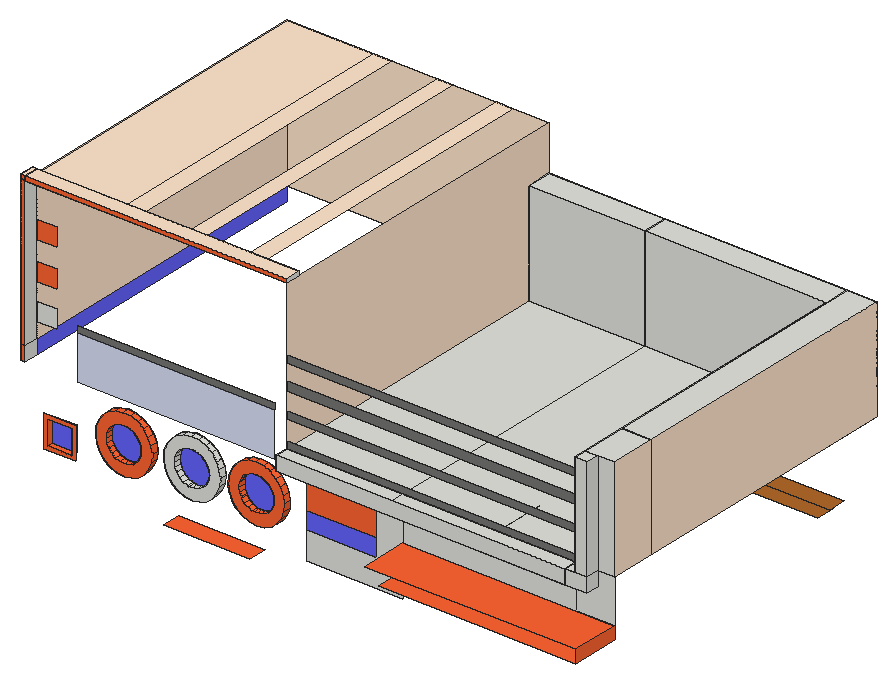
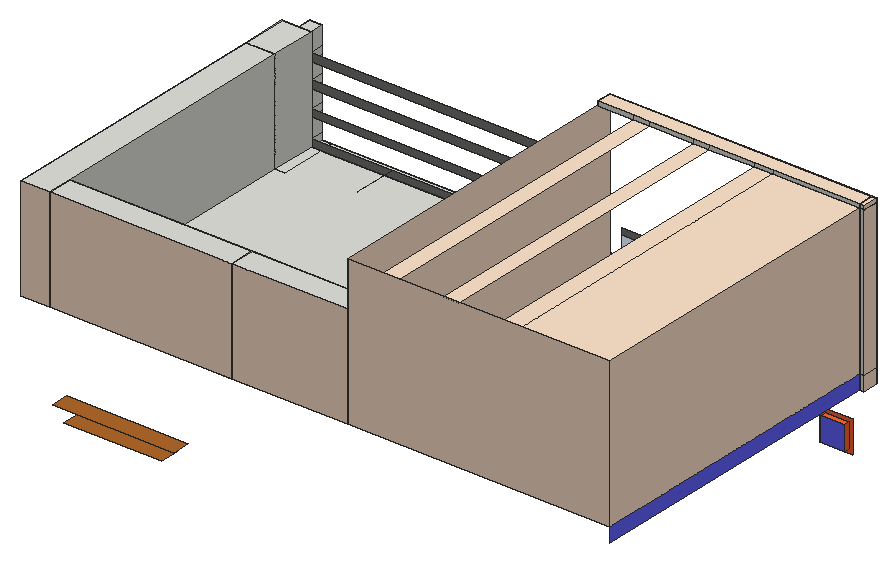
# SketchUp Ruby script. Lengths in inches.
U = 1.inch
M = Sketchup.active_model
def pt(a) = Geom::Point3d.new(a.map { |v| v * U })
def face(e, loops, mat)
  f = e.add_face(loops[0].map { |a| pt(a) })
  loops[1..].each { |l| e.add_face(l.map { |a| pt(a) }).erase! }
  f.material = f.back_material = mat if mat
  f
end
# faces: each face lists its corners as indices into pts; further lists are holes
def faces(e, pts, list, mat = nil) = list.each { |f| face(e, (f[0].is_a?(Array) ? f : [f]).map { |l| l.map { |i| pts[i] } }, mat) }
# xy, xz, yz: faces in a plane at the given z, y or x. An outline is a flat list of corners, or four numbers for a rectangle; further outlines are holes
def ring(l) = l.size == 4 ? [[l[0], l[1]], [l[2], l[1]], [l[2], l[3]], [l[0], l[3]]] : l.each_slice(2).to_a
def flat(e, list, mat, &to3) = list.each { |f| face(e, (f[0].is_a?(Array) ? f : [f]).map { |l| ring(l).map { |u, v| to3.(u, v) } }, mat) }
def xy(e, z, list, mat = nil) = flat(e, list, mat) { |x, y| [x, y, z] }
def xz(e, y, list, mat = nil) = flat(e, list, mat) { |x, z| [x, y, z] }
def yz(e, x, list, mat = nil) = flat(e, list, mat) { |y, z| [x, y, z] }
def lines(e, pts, list) = list.each { |a, b| e.add_line(pt(pts[a]), pt(pts[b])) }
# prism: a flat outline (further loops are holes) pulled along v
def prism(e, loops, v, mat = nil)
  f = face(e, loops, mat); d = Geom::Vector3d.new(v.map { |x| x * U })
  f.pushpull(f.normal.samedirection?(d) ? d.length : -d.length)
end
def box(e, o, s, mat = nil) = prism(e, [[o, [o[0] + s[0], o[1], o[2]], [o[0] + s[0], o[1] + s[1], o[2]], [o[0], o[1] + s[1], o[2]]]], [0, 0, s[2]], mat)
def at(x, y, z, deg = 0) = Geom::Transformation.translation(pt([x, y, z])) * Geom::Transformation.rotation(ORIGIN, Z_AXIS, deg.degrees)
def axes(o, x, y, z) = Geom::Transformation.new([*x, 0, *y, 0, *z, 0, *pt(o).to_a, 1])
def part(name) = M.definitions.add(name)
# library, detail: a bought-in or finely detailed component or shape, given as its bounding box
def library(name, o, s) = part(name).tap { |d| box(d.entities, o, s) }
def detail(e, o, s) = box(e.add_group.entities, o, s)
def put(e, d, t, mat = nil) = e.add_instance(d, t).tap { |i| i.material = mat if mat }
def group(e, t, mat = nil) = e.add_group.tap { |g| g.transformation = t; g.material = mat if mat }.entities
root = M.entities
M.materials.add("[Color B04]").color = [255, 101, 50]
M.materials.add("[Color C01]").color = [255, 229, 204]
M.materials.add("[Color I03]").color = [101, 101, 255]
M.materials.add("[Metal Seamed]").color = [118, 119, 115]
M.materials.add("[Translucent Glass Sky Reflection]").color = [126, 138, 183]
M.materials["[Translucent Glass Sky Reflection]"].alpha = 0.52
M.materials.add("[Wood Bamboo]").color = [177, 105, 43]
xy(root,203.96,[[68.34,47.27,99.83,54.15]],"[Color B04]")
xy(root,204,[[176.05,167.4,212.05,174.15]],"[Wood Bamboo]")
xy(root,208.17,[[171.88,167.4,216.22,174.15]],"[Wood Bamboo]")
xy(root,210.04,[[20.16,54.15,29.03,56.4]],"[Color B04]")
xy(root,218.92,[[20.16,54.15,29.03,56.4]],"[Color B04]")
xy(root,219.21,[[155.5625,36.65,228,54.15]],"[Color B04]")
xy(root,223.92,[[150.6,36.65,228,54.15]],"[Color B04]")
xy(root,234.75,[[108,49.15,213.875,54.15],[213.875,49.15,222.0625,54.15],[10.25,54.15,12,59.71]])
xy(root,240,[[108,49.15,150.6,54.15],[150.6,49.15,213.875,54.15],[213.875,49.15,217.32,54.15],[217.32,49.15,222.0625,54.15],[10.25,54.15,12,59.71],
  [108,54.15,150.6,164.8],[150.6,54.15,213.875,54.15,213.875,70.82,217.32,70.82,217.32,164.8,150.6,164.8],[213.875,54.15,217.32,70.82],[217.32,54.15,228,70.82],[217.32,70.82,228,174.15],
  [108,164.8,150.6,174.15],[150.6,164.8,217.32,174.15]])
xy(root,277.75,[[217.32,49.15,222.0625,54.15],[217.32,54.15,228,70.82],[217.32,70.82,228,174.15],[108,164.8,150.6,174.15],[150.6,164.8,217.32,174.15]])
xy(root,294.3125,[[10.25,54.15,12,59.71],[12,54.15,108,59.71]])
xy(root,294.3125,[[12,59.71,43.78,174.15],[43.78,59.71,50.45,174.15],[67.12,59.71,72.65,174.15],[88.83,59.71,94.67,174.15]],"[Color C01]")
xy(root,294.4375,[[10.25,54.15,12,59.71]])
xy(root,295.8125,[[10.25,54.15,12,59.71],[12,54.15,108,59.71]],"[Color C01]")
xz(root,49.15,[[108,234.75,213.875,240],[213.875,234.75,222.0625,240],[217.32,240,222.0625,277.75]])
xz(root,51.77,[[[75.3,212.51,77.99,212.92,80.49,214.02,82.61,215.73,82.63,215.75,84.22,217.92,85.21,220.46,85.51,223.17,85.09,225.86,84.01,228.32,84,228.36,82.29,230.48,80.09,232.09,77.55,233.08,74.85,233.38,72.15,232.96,69.66,231.87,67.53,230.16,65.92,227.96,64.93,225.42,64.64,222.71,65.05,220.02,66.15,217.53,67.86,215.4,70.05,213.79,72.59,212.8],[75.07,216.57,74.07,216.7,73.42,216.79,71.89,217.42,70.57,218.44,69.55,219.76,68.92,221.29,68.7,222.94,68.92,224.59,69.55,226.13,70.57,227.45,71.89,228.46,73.42,229.1,75.07,229.32,75.46,229.27,76.72,229.1,78.26,228.46,79.58,227.45,79.6,227.42,80.59,226.13,81.23,224.59,81.45,222.94,81.23,221.29,80.59,219.76,79.58,218.44,78.49,217.59,78.26,217.42,76.72,216.79]]])
xz(root,51.77,[[[50.34,211.64,53.03,212.05,55.53,213.15,57.65,214.86,59.26,217.05,60.25,219.59,60.55,222.3,60.13,225,59.03,227.49,57.33,229.61,55.13,231.23,52.59,232.21,49.88,232.51,47.1875,232.09,44.7,231,42.57,229.29,40.96,227.09,39.97,224.55,39.68,221.85,40.09,219.15,41.1875,216.66,42.89,214.53,45.09,212.92,47.63,211.94],[50.11,215.7,48.46,215.92,46.92,216.55,45.6,217.57,44.59,218.89,43.95,220.42,43.74,222.07,43.95,223.72,44.59,225.26,45.6,226.58,46.92,227.59,48.46,228.23,50.11,228.45,51.76,228.23,53.3,227.59,54.62,226.58,55.63,225.26,56.27,223.72,56.49,222.07,56.27,220.42,55.63,218.89,54.62,217.57,53.3,216.55,51.76,215.92]],[[98.99,212.51,101.68,212.92,104.18,214.02,106.3,215.73,106.32,215.75,107.91,217.92,108.9,220.46,109.2,223.17,108.78,225.86,107.7,228.32,107.68,228.36,105.98,230.48,103.78,232.09,101.24,233.08,98.53,233.38,95.84,232.96,93.35,231.87,91.22,230.16,90.54,229.23,89.61,227.96,88.62,225.42,88.59,225.13,88.33,222.71,88.74,220.02,88.88,219.71,89.84,217.53,91.24,215.79,91.54,215.4,93.74,213.79,96.28,212.8],[98.76,216.57,97.76,216.7,97.11,216.79,95.57,217.42,94.25,218.44,93.24,219.76,93.19,219.89,92.6,221.29,92.39,222.94,92.6,224.59,92.9,225.31,93.24,226.13,94.25,227.45,95.57,228.46,97.11,229.1,98.76,229.32,99.14,229.27,100.41,229.1,101.95,228.46,103.27,227.45,103.29,227.42,104.28,226.13,104.92,224.59,105.14,222.94,104.92,221.29,104.28,219.76,103.27,218.44,101.95,217.42,100.41,216.79]]],"[Color B04]")
xz(root,54.15,[[115.2,205.5625,150.6,205.5625,150.6,234.75,140.95,234.75,140.95,215.85,115.2,215.85],[[50.34,211.64,47.63,211.94,45.09,212.92,42.89,214.53,41.1875,216.66,40.09,219.15,39.68,221.85,39.97,224.55,40.96,227.09,42.57,229.29,44.7,231,47.1875,232.09,49.88,232.51,52.59,232.21,55.13,231.23,57.33,229.61,59.03,227.49,60.13,225,60.55,222.3,60.25,219.59,59.26,217.05,57.65,214.86,55.53,213.15,53.03,212.05],[50.11,215.7,51.76,215.92,53.3,216.55,54.62,217.57,55.63,218.89,56.27,220.42,56.49,222.07,56.27,223.72,55.63,225.26,54.62,226.58,53.3,227.59,51.76,228.23,50.11,228.45,48.46,228.23,46.92,227.59,45.6,226.58,44.59,225.26,43.95,223.72,43.74,222.07,43.95,220.42,44.59,218.89,45.6,217.57,46.92,216.55,48.46,215.92]],[[75.3,212.51,72.59,212.8,70.05,213.79,67.86,215.4,66.15,217.53,65.05,220.02,64.64,222.71,64.93,225.42,65.92,227.96,67.53,230.16,69.66,231.87,72.15,232.96,74.85,233.38,77.55,233.08,80.09,232.09,82.29,230.48,84,228.36,84.01,228.32,85.09,225.86,85.51,223.17,85.21,220.46,84.22,217.92,82.63,215.75,82.61,215.73,80.49,214.02,77.99,212.92],[75.07,216.57,76.72,216.79,78.26,217.42,78.49,217.59,79.58,218.44,80.59,219.76,81.23,221.29,81.45,222.94,81.23,224.59,80.59,226.13,79.6,227.42,79.58,227.45,78.26,228.46,76.72,229.1,75.46,229.27,75.07,229.32,73.42,229.1,71.89,228.46,70.57,227.45,69.55,226.13,68.92,224.59,68.7,222.94,68.92,221.29,69.55,219.76,70.57,218.44,71.89,217.42,73.42,216.79,74.07,216.7]],[[98.99,212.51,96.28,212.8,93.74,213.79,91.54,215.4,91.24,215.79,89.84,217.53,88.88,219.71,88.74,220.02,88.33,222.71,88.59,225.13,88.62,225.42,89.61,227.96,90.54,229.23,91.22,230.16,93.35,231.87,95.84,232.96,98.53,233.38,101.24,233.08,103.78,232.09,105.98,230.48,107.68,228.36,107.7,228.32,108.78,225.86,109.2,223.17,108.9,220.46,107.91,217.92,106.32,215.75,106.3,215.73,104.18,214.02,101.68,212.92],[98.76,216.57,100.41,216.79,101.95,217.42,103.27,218.44,104.28,219.76,104.92,221.29,105.14,222.94,104.92,224.59,104.28,226.13,103.29,227.42,103.27,227.45,101.95,228.46,100.41,229.1,99.14,229.27,98.76,229.32,97.11,229.1,95.57,228.46,94.25,227.45,93.24,226.13,92.9,225.31,92.6,224.59,92.39,222.94,92.6,221.29,93.19,219.89,93.24,219.76,94.25,218.44,95.57,217.42,97.11,216.79,97.76,216.7]],[213.875,219.21,228,223.92],
  [150.6,223.92,213.875,234.75],[213.875,223.92,228,223.92,228,240,222.0625,240,222.0625,234.75,213.875,234.75],[108,234.75,150.6,240],[150.6,234.75,213.875,240],[213.875,234.75,222.0625,240],
  [217.32,240,222.0625,277.75],[222.0625,240,228,277.75],[16.84,249.64,23.47,256.26],[10.25,294.3125,12,294.4375]])
xz(root,54.15,[[[18.78,208.67,30.41,220.29],[20.16,210.04,29.03,218.92]],[115.2,222.125,140.95,234.75],[10.25,234.75,12,240],[10.25,240,12,294.3125],[16.84,262.7,23.47,269.33],
  [16.84,276.58,23.47,283.2],[12,294.3125,108,295.8125],[10.25,294.4375,12,295.8125]],"[Color B04]")
xz(root,54.15,[[50.11,215.7,51.76,215.92,53.3,216.55,54.62,217.57,55.63,218.89,56.27,220.42,56.49,222.07,56.27,223.72,55.63,225.26,54.62,226.58,53.3,227.59,51.76,228.23,50.11,228.45,48.46,228.23,46.92,227.59,45.6,226.58,44.59,225.26,43.95,223.72,43.74,222.07,43.95,220.42,44.59,218.89,45.6,217.57,46.92,216.55,48.46,215.92],[115.2,215.85,140.95,222.125],[75.07,216.57,76.72,216.79,78.26,217.42,78.49,217.59,79.58,218.44,80.59,219.76,81.23,221.29,81.45,222.94,81.23,224.59,80.59,226.13,79.6,227.42,79.58,227.45,78.26,228.46,76.72,229.1,75.46,229.27,75.07,229.32,73.42,229.1,71.89,228.46,70.57,227.45,69.55,226.13,68.92,224.59,68.7,222.94,68.92,221.29,69.55,219.76,70.57,218.44,71.89,217.42,73.42,216.79,74.07,216.7],[98.76,216.57,100.41,216.79,101.95,217.42,103.27,218.44,104.28,219.76,104.92,221.29,105.14,222.94,104.92,224.59,104.28,226.13,103.29,227.42,103.27,227.45,101.95,228.46,100.41,229.1,99.14,229.27,98.76,229.32,97.11,229.1,95.57,228.46,94.25,227.45,93.24,226.13,92.9,225.31,92.6,224.59,92.39,222.94,92.6,221.29,93.19,219.89,93.24,219.76,94.25,218.44,95.57,217.42,97.11,216.79,97.76,216.7]],"[Color I03]")
xz(root,54.15,[[108,240,217.32,242.4375],[108,249.69,217.32,252.33],[31.45,251.04,103.62,253.35],[108,258.84,217.32,262.08],[108,267.99,217.32,270.86]],"[Metal Seamed]")
xz(root,54.15,[[31.45,234.75,103.62,251.04]],"[Translucent Glass Sky Reflection]")
xz(root,56.4,[[20.16,210.04,29.03,218.92]],"[Color I03]")
xz(root,59.71,[[10.25,234.75,12,240],[10.25,240,12,294.3125],[10.25,294.3125,12,294.4375],[12,294.3125,43.78,295.8125],[43.78,294.3125,50.45,295.8125],
  [50.45,294.3125,67.12,295.8125],[67.12,294.3125,72.65,295.8125],[72.65,294.3125,88.83,295.8125],[88.83,294.3125,94.67,295.8125],[94.67,294.3125,108,295.8125],
  [10.25,294.4375,12,295.8125]])
xz(root,70.82,[[217.32,240,228,277.75]])
xz(root,164.8,[[108,240,150.6,277.75],[150.6,240,217.32,277.75]])
xz(root,174.15,[[12,240,108,294.3125],[108,240,150.6,277.75],[150.6,240,217.32,277.75],[217.32,240,228,277.75]],"[Color C01]")
yz(root,10.25,[[54.15,294.3125,59.71,294.4375]])
yz(root,10.25,[[54.15,234.75,59.71,240],[54.15,240,59.71,294.3125],[54.15,294.4375,59.71,295.8125]],"[Color C01]")
yz(root,12,[[54.15,234.75,59.71,240],[54.15,240,59.71,294.3125],[54.15,294.3125,59.71,294.4375],[54.15,294.4375,59.71,295.8125]])
yz(root,12,[[59.71,240,174.15,294.3125]],"[Color C01]")
yz(root,12,[[59.71,234.75,174.15,240]],"[Color I03]")
yz(root,20.16,[[54.15,210.04,56.4,218.92]],"[Color B04]")
yz(root,29.03,[[54.15,210.04,56.4,218.92]],"[Color B04]")
yz(root,108,[[49.15,234.75,54.15,240],[164.8,240,174.15,277.75],[54.15,294.3125,59.71,295.8125]])
yz(root,108,[[54.15,240,164.8,240,164.8,277.75,174.15,277.75,174.15,294.3125,54.15,294.3125]],"[Color C01]")
yz(root,150.6,[[164.8,240,174.15,277.75]])
yz(root,213.875,[[49.15,234.75,54.15,240]])
yz(root,217.32,[[49.15,240,54.15,242.4375],[54.15,240,70.82,277.75],[70.82,240,164.8,277.75],[164.8,240,174.15,277.75],[49.15,242.4375,54.15,249.69],
  [49.15,249.69,54.15,252.33],[49.15,252.33,54.15,258.84],[49.15,258.84,54.15,262.08],[49.15,262.08,54.15,267.99],[49.15,267.99,54.15,270.86],
  [49.15,270.86,54.15,277.75]])
yz(root,222.0625,[[49.15,234.75,54.15,240],[49.15,240,54.15,277.75]])
yz(root,228,[[36.65,219.21,54.15,223.92]],"[Color B04]")
yz(root,228,[[54.15,240,70.82,277.75],[70.82,240,174.15,277.75]],"[Color C01]")
p = [[47.63,54.15,211.94],[50.34,54.15,211.64],[50.34,51.77,211.64],[47.63,51.77,211.94],[53.03,54.15,212.05],[53.03,51.77,212.05],
  [45.09,54.15,212.92],[45.09,51.77,212.92],[55.53,54.15,213.15],[55.53,51.77,213.15],[72.59,54.15,212.8],[75.3,54.15,212.51],
  [75.3,51.77,212.51],[72.59,51.77,212.8],[77.99,54.15,212.92],[77.99,51.77,212.92],[96.28,54.15,212.8],[98.99,54.15,212.51],
  [98.99,51.77,212.51],[96.28,51.77,212.8],[101.68,54.15,212.92],[101.68,51.77,212.92],[70.05,54.15,213.79],[70.05,51.77,213.79],
  [93.74,54.15,213.79],[93.74,51.77,213.79],[42.89,54.15,214.53],[42.89,51.77,214.53],[80.49,54.15,214.02],[80.49,51.77,214.02],
  [104.18,54.15,214.02],[104.18,51.77,214.02],[57.65,54.15,214.86],[57.65,51.77,214.86],[67.86,54.15,215.4],[67.86,51.77,215.4],
  [91.54,54.15,215.4],[91.54,51.77,215.4],[82.61,54.15,215.73],[82.61,51.77,215.73],[106.3,54.15,215.73],[106.3,51.77,215.73],
  [41.1875,54.15,216.66],[41.1875,51.77,216.66],[59.26,54.15,217.05],[59.26,51.77,217.05],[66.15,54.15,217.53],[66.15,51.77,217.53],
  [91.24,54.15,215.79],[91.24,51.77,215.79],[50.11,54.15,215.7],[48.46,54.15,215.92],[48.46,51.77,215.92],[50.11,51.77,215.7],
  [51.76,54.15,215.92],[51.76,51.77,215.92],[82.63,54.15,215.75],[82.63,51.77,215.75],[84.22,54.15,217.92],[84.22,51.77,217.92],
  [106.32,54.15,215.75],[106.32,51.77,215.75],[107.91,54.15,217.92],[107.91,51.77,217.92],[89.84,54.15,217.53],[89.84,51.77,217.53],
  [46.92,54.15,216.55],[46.92,51.77,216.55],[53.3,54.15,216.55],[53.3,51.77,216.55],[45.6,54.15,217.57],[45.6,51.77,217.57],
  [54.62,54.15,217.57],[54.62,51.77,217.57],[75.07,54.15,216.57],[74.07,54.15,216.7],[74.07,51.77,216.7],[75.07,51.77,216.57],
  [76.72,54.15,216.79],[76.72,51.77,216.79],[98.76,54.15,216.57],[97.76,54.15,216.7],[97.76,51.77,216.7],[98.76,51.77,216.57],
  [100.41,54.15,216.79],[100.41,51.77,216.79],[40.09,54.15,219.15],[40.09,51.77,219.15],[73.42,54.15,216.79],[73.42,51.77,216.79],
  [97.11,54.15,216.79],[97.11,51.77,216.79],[71.89,54.15,217.42],[71.89,51.77,217.42],[78.26,54.15,217.42],[78.26,51.77,217.42],
  [95.57,54.15,217.42],[95.57,51.77,217.42],[101.95,54.15,217.42],[101.95,51.77,217.42],[60.25,54.15,219.59],[60.25,51.77,219.59],
  [70.57,54.15,218.44],[70.57,51.77,218.44],[78.49,54.15,217.59],[78.49,51.77,217.59],[94.25,54.15,218.44],[94.25,51.77,218.44],
  [102.17,54.15,217.59],[102.17,51.77,217.59],[65.05,54.15,220.02],[65.05,51.77,220.02],[88.88,54.15,219.71],[88.88,51.77,219.71],
  [44.59,54.15,218.89],[44.59,51.77,218.89],[55.63,54.15,218.89],[55.63,51.77,218.89],[79.58,54.15,218.44],[79.58,51.77,218.44],
  [103.27,54.15,218.44],[103.27,51.77,218.44],[85.21,54.15,220.46],[85.21,51.77,220.46],[108.9,54.15,220.46],[108.9,51.77,220.46],
  [69.55,54.15,219.76],[69.55,51.77,219.76],[80.59,54.15,219.76],[80.59,51.77,219.76],[93.24,54.15,219.76],[93.24,51.77,219.76],
  [104.28,54.15,219.76],[104.28,51.77,219.76],[43.95,54.15,220.42],[43.95,51.77,220.42],[56.27,54.15,220.42],[56.27,51.77,220.42],
  [39.68,54.15,221.85],[39.68,51.77,221.85],[60.55,54.15,222.3],[60.55,51.77,222.3],[88.74,54.15,220.02],[88.74,51.77,220.02],
  [68.92,54.15,221.29],[68.92,51.77,221.29],[81.23,54.15,221.29],[81.23,51.77,221.29],[93.19,54.15,219.89],[93.19,51.77,219.89],
  [104.92,54.15,221.29],[104.92,51.77,221.29],[92.6,54.15,221.29],[92.6,51.77,221.29],[64.64,54.15,222.71],[64.64,51.77,222.71],
  [88.33,54.15,222.71],[88.33,51.77,222.71],[43.74,54.15,222.07],[43.74,51.77,222.07],[56.49,54.15,222.07],[56.49,51.77,222.07],
  [85.51,54.15,223.17],[85.51,51.77,223.17],[109.2,54.15,223.17],[109.2,51.77,223.17],[68.7,54.15,222.94],[68.7,51.77,222.94],
  [81.45,54.15,222.94],[81.45,51.77,222.94],[92.39,54.15,222.94],[92.39,51.77,222.94],[105.14,54.15,222.94],[105.14,51.77,222.94],
  [39.97,54.15,224.55],[39.97,51.77,224.55],[43.95,54.15,223.72],[43.95,51.77,223.72],[56.27,54.15,223.72],[56.27,51.77,223.72],
  [60.13,54.15,225],[60.13,51.77,225],[64.93,54.15,225.42],[64.93,51.77,225.42],[88.59,54.15,225.13],[88.59,51.77,225.13],
  [68.92,54.15,224.59],[68.92,51.77,224.59],[81.23,54.15,224.59],[81.23,51.77,224.59],[92.6,54.15,224.59],[92.6,51.77,224.59],
  [104.92,54.15,224.59],[104.92,51.77,224.59],[85.09,54.15,225.86],[85.09,51.77,225.86],[108.78,54.15,225.86],[108.78,51.77,225.86],
  [44.59,54.15,225.26],[44.59,51.77,225.26],[55.63,54.15,225.26],[55.63,51.77,225.26],[40.96,54.15,227.09],[40.96,51.77,227.09],
  [69.55,54.15,226.13],[69.55,51.77,226.13],[80.59,54.15,226.13],[80.59,51.77,226.13],[92.9,54.15,225.31],[92.9,51.77,225.31],
  [104.28,54.15,226.13],[104.28,51.77,226.13],[59.03,54.15,227.49],[59.03,51.77,227.49],[88.62,54.15,225.42],[88.62,51.77,225.42],
  [45.6,54.15,226.58],[45.6,51.77,226.58],[54.62,54.15,226.58],[54.62,51.77,226.58],[93.24,54.15,226.13],[93.24,51.77,226.13],
  [65.92,54.15,227.96],[65.92,51.77,227.96],[89.61,54.15,227.96],[89.61,51.77,227.96],[84.01,54.15,228.32],[84.01,51.77,228.32],
  [107.7,54.15,228.32],[107.7,51.77,228.32],[70.57,54.15,227.45],[70.57,51.77,227.45],[79.6,54.15,227.42],[79.6,51.77,227.42],
  [94.25,54.15,227.45],[94.25,51.77,227.45],[103.29,54.15,227.42],[103.29,51.77,227.42],[46.92,54.15,227.59],[46.92,51.77,227.59],
  [53.3,54.15,227.59],[53.3,51.77,227.59],[42.57,54.15,229.29],[42.57,51.77,229.29],[79.58,54.15,227.45],[79.58,51.77,227.45],
  [103.27,54.15,227.45],[103.27,51.77,227.45],[57.33,54.15,229.61],[57.33,51.77,229.61],[71.89,54.15,228.46],[71.89,51.77,228.46],
  [78.26,54.15,228.46],[78.26,51.77,228.46],[95.57,54.15,228.46],[95.57,51.77,228.46],[101.95,54.15,228.46],[101.95,51.77,228.46],
  [48.46,54.15,228.23],[48.46,51.77,228.23],[51.76,54.15,228.23],[51.76,51.77,228.23],[67.53,54.15,230.16],[67.53,51.77,230.16],
  [90.54,54.15,229.23],[90.54,51.77,229.23],[50.11,54.15,228.45],[50.11,51.77,228.45],[84,54.15,228.36],[84,51.77,228.36],
  [107.68,54.15,228.36],[107.68,51.77,228.36],[82.29,54.15,230.48],[82.29,51.77,230.48],[105.98,54.15,230.48],[105.98,51.77,230.48],
  [73.42,54.15,229.1],[73.42,51.77,229.1],[76.72,54.15,229.1],[76.72,51.77,229.1],[97.11,54.15,229.1],[97.11,51.77,229.1],
  [100.41,54.15,229.1],[100.41,51.77,229.1],[75.07,54.15,229.32],[75.07,51.77,229.32],[75.46,54.15,229.27],[75.46,51.77,229.27],
  [98.76,54.15,229.32],[98.76,51.77,229.32],[99.14,54.15,229.27],[99.14,51.77,229.27],[91.22,54.15,230.16],[91.22,51.77,230.16],
  [44.7,54.15,231],[44.7,51.77,231],[55.13,54.15,231.23],[55.13,51.77,231.23],[69.66,54.15,231.87],[69.66,51.77,231.87],
  [93.35,54.15,231.87],[93.35,51.77,231.87],[80.09,54.15,232.09],[80.09,51.77,232.09],[103.78,54.15,232.09],[103.78,51.77,232.09],
  [47.1875,54.15,232.09],[47.1875,51.77,232.09],[52.59,54.15,232.21],[52.59,51.77,232.21],[72.15,54.15,232.96],[72.15,51.77,232.96],
  [95.84,54.15,232.96],[95.84,51.77,232.96],[49.88,54.15,232.51],[49.88,51.77,232.51],[77.55,54.15,233.08],[77.55,51.77,233.08],
  [101.24,54.15,233.08],[101.24,51.77,233.08],[74.85,54.15,233.38],[74.85,51.77,233.38],[98.53,54.15,233.38],[98.53,51.77,233.38],
  [187.9,54.15,242.4375],[187.9,69.96,242.4375]]
faces(root,p,[[0,1,2,3],[1,4,5,2],[6,0,3,7],[4,8,9,5],[16,17,18,19],[17,20,21,18],[24,16,19,25],[26,6,7,27],
  [20,30,31,21],[8,32,33,9],[36,24,25,37],[30,40,41,31],[42,26,27,43],[32,44,45,33],[48,36,37,49],[50,51,52,53],
  [54,50,53,55],[40,60,61,41],[60,62,63,61],[64,48,49,65],[51,66,67,52],[68,54,55,69],[66,70,71,67],[72,68,69,73],
  [80,81,82,83],[84,80,83,85],[86,42,43,87],[81,90,91,82],[90,96,97,91],[98,84,85,99],[44,100,101,45],[96,106,107,97],
  [108,98,99,109],[112,64,65,113],[70,114,115,71],[116,72,73,117],[120,108,109,121],[62,124,125,63],[106,130,131,107],[132,120,121,133],
  [114,134,135,115],[136,116,117,137],[138,86,87,139],[100,140,141,101],[142,112,113,143],[130,148,149,131],[150,132,133,151],[148,152,153,149],
  [156,142,143,157],[134,158,159,135],[160,136,137,161],[124,164,165,125],[152,170,171,153],[172,150,151,173],[174,138,139,175],[158,176,177,159],
  [178,160,161,179],[140,180,181,141],[184,156,157,185],[170,190,191,171],[192,172,173,193],[164,196,197,165],[176,198,199,177],[200,178,179,201],
  [202,174,175,203],[190,208,209,191],[210,192,193,211],[180,212,213,181],[214,184,185,215],[198,216,217,199],[218,200,201,219],[208,220,221,209],
  [224,214,215,225],[196,228,229,197],[220,234,235,221],[236,210,211,237],[216,238,239,217],[240,218,219,241],[242,202,203,243],[246,236,237,247],
  [212,248,249,213],[234,254,255,235],[256,246,247,257],[238,258,259,239],[260,240,241,261],[264,224,225,265],[258,266,267,259],[266,260,261,267],
  [228,270,271,229],[270,274,275,271],[254,280,281,255],[282,256,257,283],[280,288,289,281],[290,282,283,291],[292,264,265,293],[294,242,243,295],
  [288,290,291,289],[248,296,297,249],[300,292,293,301],[274,304,305,275],[306,294,295,307],[296,308,309,297],[312,300,301,313],[314,306,307,315],
  [304,318,319,305],[308,314,315,309],[322,312,313,323],[318,322,323,319]],"[Color B04]")
faces(root,p,[[10,11,12,13],[11,14,15,12],[22,10,13,23],[14,28,29,15],[34,22,23,35],[28,38,39,29],[46,34,35,47],[38,56,57,39],
  [56,58,59,57],[74,75,76,77],[78,74,77,79],[75,88,89,76],[88,92,93,89],[94,78,79,95],[92,102,103,93],[104,94,95,105],
  [110,46,47,111],[118,104,105,119],[58,122,123,59],[102,126,127,103],[128,118,119,129],[126,144,145,127],[146,128,129,147],[154,110,111,155],
  [122,162,163,123],[144,166,167,145],[168,146,147,169],[182,154,155,183],[166,186,187,167],[188,168,169,189],[162,194,195,163],[186,204,205,187],
  [206,188,189,207],[222,182,183,223],[194,226,227,195],[204,230,231,205],[232,206,207,233],[244,232,233,245],[230,250,251,231],[252,244,245,253],
  [262,222,223,263],[226,268,269,227],[268,272,273,269],[250,276,277,251],[278,252,253,279],[276,284,285,277],[286,278,279,287],[284,286,287,285],
  [298,262,263,299],[272,302,303,273],[310,298,299,311],[302,316,317,303],[320,310,311,321],[316,320,321,317]])
lines(root,p,[[324,325]])
